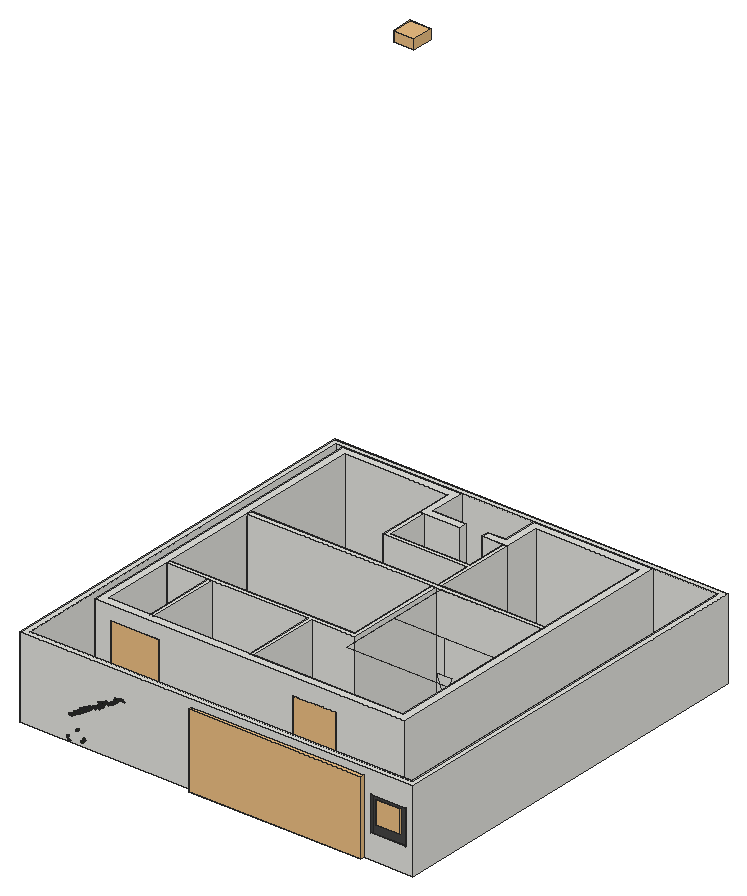
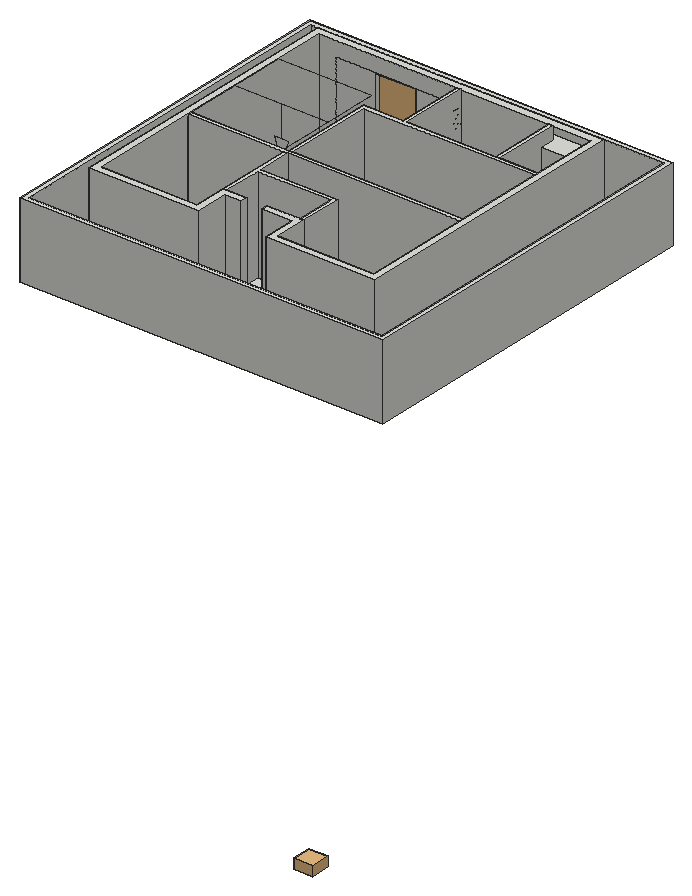
# SketchUp Ruby script. Lengths in millimetres.
U = 1.mm
M = Sketchup.active_model
def pt(a) = Geom::Point3d.new(a.map { |v| v * U })
def face(e, loops, mat)
  f = e.add_face(loops[0].map { |a| pt(a) })
  loops[1..].each { |l| e.add_face(l.map { |a| pt(a) }).erase! }
  f.material = f.back_material = mat if mat
  f
end
# faces: each face lists its corners as indices into pts; further lists are holes
def faces(e, pts, list, mat = nil) = list.each { |f| face(e, (f[0].is_a?(Array) ? f : [f]).map { |l| l.map { |i| pts[i] } }, mat) }
# xy, xz, yz: faces in a plane at the given z, y or x. An outline is a flat list of corners, or four numbers for a rectangle; further outlines are holes
def ring(l) = l.size == 4 ? [[l[0], l[1]], [l[2], l[1]], [l[2], l[3]], [l[0], l[3]]] : l.each_slice(2).to_a
def flat(e, list, mat, &to3) = list.each { |f| face(e, (f[0].is_a?(Array) ? f : [f]).map { |l| ring(l).map { |u, v| to3.(u, v) } }, mat) }
def xy(e, z, list, mat = nil) = flat(e, list, mat) { |x, y| [x, y, z] }
def xz(e, y, list, mat = nil) = flat(e, list, mat) { |x, z| [x, y, z] }
def yz(e, x, list, mat = nil) = flat(e, list, mat) { |y, z| [x, y, z] }
def lines(e, pts, list) = list.each { |a, b| e.add_line(pt(pts[a]), pt(pts[b])) }
# prism: a flat outline (further loops are holes) pulled along v
def prism(e, loops, v, mat = nil)
  f = face(e, loops, mat); d = Geom::Vector3d.new(v.map { |x| x * U })
  f.pushpull(f.normal.samedirection?(d) ? d.length : -d.length)
end
def box(e, o, s, mat = nil) = prism(e, [[o, [o[0] + s[0], o[1], o[2]], [o[0] + s[0], o[1] + s[1], o[2]], [o[0], o[1] + s[1], o[2]]]], [0, 0, s[2]], mat)
def at(x, y, z, deg = 0) = Geom::Transformation.translation(pt([x, y, z])) * Geom::Transformation.rotation(ORIGIN, Z_AXIS, deg.degrees)
def axes(o, x, y, z) = Geom::Transformation.new([*x, 0, *y, 0, *z, 0, *pt(o).to_a, 1])
def part(name) = M.definitions.add(name)
# library, detail: a bought-in or finely detailed component or shape, given as its bounding box
def library(name, o, s) = part(name).tap { |d| box(d.entities, o, s) }
def detail(e, o, s) = box(e.add_group.entities, o, s)
def put(e, d, t, mat = nil) = e.add_instance(d, t).tap { |i| i.material = mat if mat }
def group(e, t, mat = nil) = e.add_group.tap { |g| g.transformation = t; g.material = mat if mat }.entities
root = M.entities
M.materials.add("[Granite Dark Gray]").color = [69, 68, 68]
M.materials.add("efeu1").color = [18, 25, 13]
M.materials.add("efeu2").color = [43, 57, 29]
c1 = part("ivyleaf_10")
p = [[0,12.8,-0.8],[-1.5,51.3,-10.9],[-4.9,51,-11.6],[-13.6,26.5,-7.3],[-13.2,15.9,-4.6],[-21.1,19.3,-7.2],
  [-29.5,16.3,-8.3],[-29.2,8.3,-6.2],[-19.7,-9.8,0.5],[-7.6,-13,4],[1,-12.2,5.8],[-0.4,51.1,-11.1],
  [-1.5,51.1,-10.9],[1,-12.4,5.9],[16.9,-12.4,3.5],[35.1,9.1,-5.1],[35,12.9,-6.1],[20.5,16.4,-4.9],
  [15.8,15,-3.8],[15.3,27.6,-7.1],[12.8,31.3,-7.8]]
faces(c1.entities,p,[[0,1,2,3,4,5,6,7,8,9,10],[11,12,0,13,14,15,16,17,18,19,20]],"efeu2")
c2 = part("ivyleaf_9")
p = [[39.1,54.8,31.7],[34.5,51.8,30.2],[-5.3,25.2,17.3],[-17.9,28.3,20.9],[-21.6,21.7,17],[-20.2,4.3,5.3],
  [-22.9,-0.3,2.5],[-17.1,-4,-0.6],[-2,-2.1,-1.2],[-0.7,-15.4,-10.1],[16.6,-22.3,-16.7],[21.1,-15.1,-12.5],
  [32.7,-10.7,-11],[46.1,-1.8,-6.6],[30.8,11.2,3.8]]
faces(c2.entities,p,[[0,1,2,3,4,5,6,7,8,9,10,11,12,13,14]],"efeu1")
c3 = library("portao terminado by jhon",[0,-102.4,0],[4575,189.4,2762])
c4 = library("Group\#11",[0,0,0],[1682.8,214.9,2070.1])
c5 = library("ITDHP",[-33.4,-34.2,-15.9],[968.5,150,1668.6])
c6 = part("Group242\#1")
p = [[0,0,0],[0,0,-997.2],[-228.7,0,-997.2],[1488.8,-1739.7,0],[-1488.8,-1739.7,0],[1488.8,1739.7,0],
  [1488.8,0,0],[-1488.8,1739.7,0],[228.7,0,-997.2],[-1488.8,0,0],[0,0,-1614.2]]
lines(c6.entities,p,[[0,1],[1,2],[3,4],[5,6],[7,5],[1,8],[9,0],[0,6],[8,10],[4,9],[6,3],[2,10],
  [9,7]])
c7 = part("Rectangle Light\#3")
put(c7.entities,c6,at(0,0,0))
c8 = part("Group\#23")
box(c8.entities,[0,0,0],[9144,9144,101.6])
c9 = library("RAGHU   344B",[7.3,0,0],[307,195.6,25.4])
c10 = library("Dome Light\#2",[-304.8,-304.8,0],[609.6,609.6,304.8])
p = [[3261.9,2460,2644.4],[3261.9,2460,376.2],[1860.6,2460,376.2],[1860.6,2460,2644.4]]
lines(root,p,[[0,1],[2,3],[1,2]])
put(root,c1,axes([2087.5,1125.2,996.5],[1.14647,-0.14425,0.30188],[0.61451,0.08776,-0.60237],[0.16683,0.66806,0.14431]))
put(root,c1,axes([2227,1123.5,1076.7],[-1.14042,-0.39726,-0.06521],[0.10481,0.03494,-0.71894],[0.75898,-0.60174,0.0013]))
put(root,c1,axes([2487.7,1127.9,1168.1],[1.40853,-0.16077,0.0819],[0.14809,-0.0276,-0.75728],[0.30982,0.74409,-0.01039]))
put(root,c1,axes([2211.8,1127,1015.9],[1.36855,-0.00361,-0.09168],[-0.17454,-0.0063,-0.71906],[0.00529,0.72487,-0.0067]))
put(root,c1,axes([1950.7,1114.9,376.8],[0.16677,0.51977,0.47683],[0.13328,0.47171,-0.52706],[-1.3358,0.11196,0.00694]))
put(root,c2,axes([2675.6,1112.7,1367.7],[1.14223,0.42917,0.21801],[0.26909,0.1759,-0.73551],[-0.87572,0.61383,0.05835]))
put(root,c1,axes([1941.5,1127.4,839.5],[1.08139,-0.33434,0.00262],[0.02934,0.02105,-0.65876],[0.63567,0.56781,0.02596]))
put(root,c2,axes([2938.7,1117.8,1436.5],[1.15383,-0.02714,0.55158],[1.03903,0.15292,-0.59253],[-0.15844,0.80524,0.13112]))
put(root,c1,axes([1802.2,1127.3,748.7],[0.87541,-0.43119,-0.08942],[-0.10174,0.07367,-0.63024],[0.83191,0.46275,0.01702]))
put(root,c2,axes([2883.8,1117.5,1403.4],[1.44406,0.20956,0.20212],[0.37338,0.04888,-0.78715],[-0.40943,0.78369,-0.00495]))
put(root,c1,axes([2734.2,1124.8,1338.8],[-1.44401,-0.1281,-0.03694],[0.06469,0.02052,-0.76933],[0.24534,-0.75935,-0.01456]))
put(root,c1,axes([2138.7,1124.5,1019.4],[-0.75397,0.57073,-0.00023],[-0.00302,-0.00138,-0.69474],[-1.0862,-0.39616,0.00209]))
put(root,c1,axes([2245.3,1130.3,1039.4],[1.22175,0.24323,-0.15892],[-0.26862,-0.07583,-0.68618],[-0.48334,0.65696,-0.02036]))
put(root,c1,axes([2785.2,1124,1392.8],[0.87594,-0.48565,-0.40345],[-0.39684,0.35434,-0.6644],[1.13421,0.49904,0.07912]))
put(root,c1,axes([2595.6,1124.3,1225.1],[-1.31814,0.24129,0.24295],[-0.45087,0.05814,-0.73309],[-0.47053,-0.73166,0.02186]))
put(root,c1,axes([2418,1128.8,1162.7],[-1.16783,0.29379,-0.26503],[0.40269,-0.16962,-0.67789],[-0.63632,-0.64652,0.05741]))
put(root,c1,axes([2246.2,1132.2,1063.9],[0.54559,-0.61256,0.19596],[0.57494,-0.06115,-0.63309],[1.08059,0.34182,0.2379]))
put(root,c1,axes([2113,1126,187.9],[0.80503,0.17543,0.57575],[1.01265,0.21996,-0.45792],[-0.53546,0.67972,-0.00041]))
put(root,c2,axes([2651.2,1128.9,1308.3],[-0.72724,0.20612,0.62733],[-1.14354,0.19209,-0.4291],[-0.52125,-0.70899,0.06612]))
put(root,c1,axes([2290.1,1127,1106.5],[-0.78834,0.57906,-0.04144],[0.05747,-0.02934,-0.71192],[-1.10339,-0.41525,-0.00747]))
put(root,c2,axes([2593.4,1126.5,1287.1],[1.40082,-0.25988,0.08859],[0.19166,0.01971,-0.77885],[0.48614,0.74108,0.05178]))
put(root,c1,axes([1905.8,1116.9,353.5],[-0.20645,0.19287,0.66736],[-0.6237,0.58136,-0.22129],[-1.16574,-0.3452,0.0002]))
put(root,c1,axes([2376.5,1125.8,1120.4],[0.41629,0.67018,0.1664],[0.02658,0.17022,-0.70392],[-1.31394,0.21577,0.03848]))
put(root,c1,axes([2077.2,1130.6,100.3],[-1.20166,-0.34105,0.12031],[-0.20148,-0.05716,-0.71762],[0.65815,-0.64021,-0.00002]))
put(root,c2,axes([3074.3,1117.4,1564],[-0.14401,0.62355,0.52426],[-0.5244,0.47589,-0.60579],[-1.45907,-0.23258,0.16598]))
put(root,c1,axes([2083.8,1127.2,985.5],[-0.9922,-0.29503,-0.33284],[0.58225,0.13437,-0.5983],[0.61443,-0.60375,0.02949]))
put(root,c1,axes([1847.2,1134.9,825.7],[0.26434,0.55426,-0.30055],[-0.38483,-0.25234,-0.5588],[-1.13659,0.21434,0.1193]))
put(root,c1,axes([2033.8,1132.8,966.4],[1.20012,-0.23106,-0.15832],[-0.28876,0.04606,-0.67153],[0.4481,0.64852,-0.00872]))
put(root,c2,axes([2529.7,1141.6,1158.8],[0.17517,-0.73,0.19546],[0.26456,-0.17719,-0.72723],[1.41374,0.12361,0.11187]))
put(root,c1,axes([1701.9,1128.5,6.6],[0.41838,-0.09412,-0.61048],[-1.06203,0.2476,-0.23911],[0.50409,0.59975,0.00292]))
put(root,c1,axes([2611,1128.2,1269.6],[0.17115,0.74499,0.07381],[-0.06511,0.07835,-0.74915],[-1.42331,0.086,0.04314]))
put(root,c1,axes([2156.7,1130.4,990.8],[-1.12894,-0.39996,-0.06692],[0.11408,0.0308,-0.71538],[0.7633,-0.59615,0.00794]))
put(root,c2,axes([2648.4,1126.8,1311.5],[1.39789,-0.11145,-0.17675],[-0.32698,0.04555,-0.74266],[0.22635,0.75409,0.01873]))
put(root,c1,axes([3086.7,1129.5,1527.5],[-0.87891,-0.62071,-0.33517],[0.63358,0.16142,-0.75763],[1.18365,-0.54731,0.15666]))
put(root,c1,axes([2872.3,1134.5,1396.1],[-1.18913,-0.46802,0.23312],[-0.38278,-0.12017,-0.78031],[0.91856,-0.65596,-0.02338]))
put(root,c2,axes([2527,1140.2,1184.9],[-1.4479,-0.0903,-0.02056],[0.03876,0.00287,-0.76611],[0.17195,-0.76105,-0.00045]))
put(root,c2,axes([2684.4,1124.5,1319.4],[1.0942,0.49964,-0.08552],[-0.12552,-0.05449,-0.76169],[-0.95654,0.57869,0.00212]))
put(root,c1,axes([2166.9,1133.9,982.2],[1.20048,0.27627,0.02283],[0.00864,0.04644,-0.68742],[-0.52752,0.62947,0.0407]))
put(root,c2,axes([2611.2,1131.1,1219.3],[1.29213,-0.19777,0.3143],[0.62228,0.00788,-0.70133],[0.33504,0.7481,0.09048]))
put(root,c1,axes([1641.3,1125,74.3],[0.34683,0.44503,-0.4286],[0.28466,0.40179,0.48079],[1.14094,-0.23553,0.01033]))
put(root,c1,axes([2002.9,1136.6,906.3],[-0.1027,-0.66383,0.00555],[0.02053,-0.00644,-0.66592],[1.26328,-0.05386,0.01127]))
put(root,c1,axes([2344.7,1133.8,1092.8],[-1.26781,0.26235,0.00767],[-0.08042,-0.08656,-0.70948],[-0.49299,-0.66054,0.09602]))
put(root,c2,axes([2711.4,1125.1,1339.7],[0.66533,0.6864,-0.0181],[-0.03371,-0.01129,-0.77022],[-1.30637,0.34987,0.01066]))
put(root,c1,axes([1798,1141.1,753.8],[-0.57971,-0.53097,0.24391],[-0.25724,-0.20357,-0.61196],[1.0819,-0.33291,-0.01481]))
put(root,c1,axes([1741.7,1141.3,714.9],[-0.79482,-0.37017,0.33114],[-0.4073,-0.2563,-0.55642],[0.853,-0.4673,0.04287]))
put(root,c1,axes([2265.9,1134.2,1011.5],[1.03278,-0.19104,-0.4391],[-0.69613,0.26296,-0.56643],[0.58821,0.64663,0.10062]))
put(root,c1,axes([1952.8,1141.9,831.4],[0.77305,-0.50539,0.20075],[0.36414,-0.10173,-0.64323],[0.96878,0.44152,0.08159]))
put(root,c1,axes([2042.8,1138.8,920.3],[1.13684,0.31347,-0.01678],[-0.02813,-0.00794,-0.67459],[-0.59678,0.59751,-0.00017]))
put(root,c1,axes([2092.9,1138.9,946.1],[0.83948,0.51607,-0.0565],[-0.04985,-0.05192,-0.67875],[-0.98679,0.44165,-0.01377]))
put(root,c1,axes([2204.8,1132.1,1024.1],[0.3654,0.63545,0.29134],[0.17355,0.27678,-0.66379],[-1.31907,0.21244,-0.00663]))
put(root,c1,axes([2055.9,1138.4,910.8],[-1.19265,0.24212,0.03133],[-0.14567,-0.11287,-0.65856],[-0.44123,-0.6172,0.13272]))
put(root,c1,axes([1663.3,1133.7,111.6],[0.44207,-0.21789,-0.57506],[-0.83258,0.37348,-0.31821],[0.82255,0.49513,-0.01304]))
put(root,c1,axes([2184,1137.8,965.5],[-1.33928,-0.07647,-0.06876],[0.13459,-0.01463,-0.7075],[0.14209,-0.7069,0.02208]))
put(root,c2,axes([2576.4,1144.7,1209.1],[-1.10889,0.13379,0.48618],[-0.95061,-0.05123,-0.5845],[-0.13163,-0.75711,0.12546]))
put(root,c1,axes([1961.4,1140.4,834.8],[-0.51233,-0.62282,-0.03193],[0.02408,0.02931,-0.6785],[1.18666,-0.26949,-0.00002]))
put(root,c1,axes([1861.6,1143.6,765.7],[0.11262,-0.65084,0.09162],[0.22553,-0.07991,-0.64425],[1.23039,0.07422,0.1097]))
put(root,c1,axes([2100.5,1135.7,963.8],[0.35088,-0.56899,-0.32951],[-0.03237,0.33797,-0.59313],[1.25097,0.16834,0.07707]))
put(root,c1,axes([1912.8,1138.8,840],[-0.41835,0.63903,-0.06258],[0.06384,-0.05463,-0.67563],[-1.22034,-0.22192,-0.01389]))
put(root,c1,axes([2037.2,1142.3,912.8],[0.57227,0.59214,-0.09712],[-0.05534,-0.09412,-0.6639],[-1.14067,0.30164,-0.01651]))
put(root,c2,axes([3216.3,1134.5,1584.3],[1.60333,-0.08607,0.1036],[0.21434,0.09021,-0.84085],[0.14061,0.84398,0.10044]))
put(root,c1,axes([1722.1,1142.7,720],[-0.8891,0.41506,-0.1659],[0.07984,-0.1982,-0.614],[-0.84695,-0.4544,0.11628]))
put(root,c1,axes([1683.5,1143.9,697.5],[0.99386,-0.3603,0.08583],[0.24125,0.03446,-0.6266],[0.66235,0.52809,0.09944]))
put(root,c2,axes([2651.4,1144.5,1255.4],[-1.39761,0.26588,-0.01109],[0.0257,0.00473,-0.78095],[-0.50582,-0.73442,-0.00904]))
put(root,c1,axes([1964.2,1144.3,820.5],[1.28133,-0.01571,0.05918],[0.11272,0.0013,-0.67343],[0.02957,0.67584,0.00267]))
put(root,c1,axes([2250.9,1137.8,1058.7],[0.64921,0.57335,0.2312],[0.17275,0.21475,-0.66647],[-1.16383,0.3517,0.03005]))
put(root,c1,axes([2340.8,1137.4,1100.2],[-0.18264,-0.02984,0.71109],[1.1457,0.37938,0.09716],[-0.72261,0.60904,-0.02568]))
put(root,c1,axes([2011.3,1139.5,905.1],[-0.72427,0.20234,0.54537],[-1.03186,0.11275,-0.42015],[-0.40112,-0.65539,0.09609]))
put(root,c1,axes([2924.7,1136.7,1429.1],[-0.60924,0.68131,0.32435],[-0.41882,0.25272,-0.74804],[-1.37368,-0.37922,0.08422]))
put(root,c1,axes([2433.8,1146.8,1120],[-1.05987,0.38935,-0.31691],[0.39921,-0.24955,-0.67519],[-0.86806,-0.59015,0.07643]))
put(root,c1,axes([2223.4,1143.2,989.3],[-1.00531,-0.4412,-0.21337],[0.4215,0.06495,-0.68259],[0.83205,-0.56597,0.08799]))
put(root,c1,axes([1910.2,1143.8,787],[-0.48525,-0.47153,0.39714],[0.78354,0.18966,0.48949],[-0.87334,0.43215,0.2185]))
put(root,c1,axes([2311.9,1144.4,1047.3],[-1.34262,-0.1772,0.10149],[-0.18137,-0.03717,-0.72726],[0.34374,-0.71175,0.01271]))
put(root,c1,axes([2590.6,1146,1201.5],[1.28279,0.30834,0.20555],[0.36073,0.07976,-0.74117],[-0.60603,0.70013,-0.00609]))
put(root,c1,axes([1960.7,1137.6,858.3],[0.32576,-0.02559,-0.66433],[-0.78395,0.53438,-0.12671],[0.99317,0.4302,0.11788]))
put(root,c1,axes([1982.9,1149.2,825.1],[1.28689,0.00904,0.05914],[0.11267,-0.0039,-0.67621],[-0.01649,0.67874,-0.00467]))
put(root,c1,axes([1833.5,1146.4,784],[-0.83766,0.46308,-0.00992],[0.01893,-0.00423,-0.63886],[-0.88134,-0.44023,-0.00429]))
put(root,c1,axes([2295.7,1148.4,1017.4],[0.80941,-0.58283,0.08136],[-0.11218,0.05769,0.72137],[-1.11436,-0.42914,-0.01353]))
put(root,c2,axes([2617.5,1141.4,1240.2],[1.41382,0.20155,-0.1232],[-0.2359,-0.01349,-0.76948],[-0.3827,0.75289,0.0192]))
put(root,c1,axes([3173.9,1150.6,1595.6],[1.4026,0.42686,0.03072],[0.02869,0.03524,-0.85136],[-0.814,0.73677,0.02292]))
put(root,c1,axes([2347.6,1150.4,1054.1],[0.14125,0.72377,-0.09823],[-0.51469,-0.06449,-0.67949],[-1.29131,0.10487,0.26009]))
put(root,c1,axes([1976.8,1151,841.1],[0.13058,0.67305,-0.08399],[-0.0077,-0.08401,-0.67652],[-1.29086,0.06859,-0.00446]))
put(root,c1,axes([1837.1,1161.2,758.5],[-0.6104,-0.37581,0.43332],[-0.04619,-0.48712,-0.44044],[1.09066,-0.23096,0.22386]))
put(root,c2,axes([2919,1151.2,1418.9],[1.34132,-0.40615,-0.05695],[-0.11526,0.00892,-0.81312],[0.77199,0.70701,-0.02246]))
put(root,c1,axes([2830.5,1140.4,1345.8],[0.00272,-0.01779,0.80228],[0.68542,0.71696,0.01526],[-1.36483,0.36003,0.00926]))
put(root,c1,axes([1732.9,1151.8,684.4],[-0.85829,-0.22462,-0.39564],[0.78116,0.03946,-0.49025],[0.37355,-0.59863,0.11614]))
put(root,c1,axes([3030.4,1151.4,1506],[-1.53799,0.1931,-0.06685],[0.11701,-0.03029,-0.83072],[-0.37088,-0.8103,0.01512]))
put(root,c1,axes([1774.7,1152.8,716.1],[-1.16417,0.19732,0.08542],[-0.16731,0.00557,-0.64237],[-0.37346,-0.6176,0.0215]))
put(root,c1,axes([2493.6,1155,1170.6],[-1.29549,0.31597,-0.11703],[0.1969,-0.05507,-0.75042],[-0.61029,-0.68848,0.00631]))
put(root,c1,axes([3056.5,1155.1,1512.6],[-1.57039,-0.071,-0.10658],[0.20404,-0.00285,-0.82809],[0.13331,-0.83198,0.01193]))
put(root,c1,axes([2113.4,1156.8,912.6],[1.1383,-0.03936,-0.35907],[-0.64946,0.16622,-0.58662],[0.22547,0.67751,0.12306]))
put(root,c1,axes([2048.9,1158.8,879.4],[1.28694,0.08427,-0.10291],[-0.20899,0.05281,-0.6783],[-0.14286,0.68194,0.06524]))
put(root,c1,axes([1976.3,1163.9,842.3],[-1.14856,0.29947,0.08062],[-0.16168,0.01002,-0.6731],[-0.56767,-0.60877,0.02858]))
put(root,c1,axes([1733.2,1165,691.6],[-0.60057,0.55437,-0.02515],[0.03922,-0.01721,-0.63782],[-1.05543,-0.31609,-0.00939]))
put(root,c2,axes([2574.4,1157.2,1220.3],[1.14365,0.46244,0.13789],[0.15892,0.11725,-0.75712],[-0.90455,0.60527,0.04132]))
put(root,c2,axes([2624.1,1157.6,1238.1],[0.80785,0.59559,0.25643],[0.26398,0.216,-0.73128],[-1.20557,0.4464,0.01171]))
put(root,c3,axes([5232.4,1226.8,-101.6],[1.10738,0,0],[0,1,0],[0,0,0.78614]))
put(root,c4,axes([7229.2,2446,210.4],[0.74576,0,0],[0,0.57,0],[0,0,1.13036]))
put(root,c5,axes([1909.4,2477.6,384.8],[1.44679,0,0],[0,0.92467,0],[0,0,1.35933]))
g1 = group(root,at(2833.1,2674.6,0))
xy(g1,0,[[0,0,127,2133.6]])
xy(g1,3048,[[0,0,127,2133.6]])
xz(g1,2133.6,[[0,0,127,3048]])
yz(g1,0,[[0,0,2133.6,3048]])
yz(g1,127,[[0,0,2133.6,3048]])
g2 = group(root,at(1613.9,2674.6,0))
prism(g2,[[[5562.6,5105.4,0],[5562.6,2133.6,0],[4292.6,2133.6,0],[4292.6,0,0],[4165.6,0,0],[4165.6,2133.6,0],[1346.2,2133.6,0],[1219.2,2133.6,0],[0,2133.6,0],[0,2260.6,0],[5435.6,2260.6,0],[5435.6,5105.4,0]]],[0,0,3048])
put(root,c7,at(8812,6040.4,3047.7))
put(root,c8,at(1385.3,2446,-101.6))
g3 = group(root,at(1385.3,2446,0))
xy(g3,0,[[0,0,0,9144,3500.3,9144,3500.3,8102.6,4459.1,8102.6,4459.1,7874,3276.6,7874,3276.6,8915.4,228.6,8915.4,228.6,228.6,8915.4,228.6,8915.4,8915.4,5867.4,8915.4,5867.4,7874,5119.1,7874,5119.1,8102.6,5638.8,8102.6,5638.8,9144,9144,9144,9144,0]])
xy(g3,210.4,[[5838.3,0,7098.8,228.6]])
xy(g3,288,[[4394.2,228.6,4521.2,579.4]])
xy(g3,376.3,[[475.3,0,1877,723.9]])
xy(g3,2548.8,[[5838.3,0,7098.8,228.6]])
xy(g3,2564.5,[[4394.2,228.6,4521.2,579.4]])
xy(g3,2644.4,[[475.3,0,1877,723.9]])
xy(g3,3048,[[0,0,9144,0,9144,9144,5638.8,9144,5638.8,8102.6,5119.1,8102.6,5119.1,7874,5867.4,7874,5867.4,8915.4,8915.4,8915.4,8915.4,228.6,228.6,228.6,228.6,8915.4,3276.6,8915.4,3276.6,7874,4459.1,7874,4459.1,8102.6,3500.3,8102.6,3500.3,9144,0,9144]])
xz(g3,0,[[[0,0,9144,3048],[475.3,376.3,1877,2644.4],[5838.3,210.4,7098.8,2548.8]]])
xz(g3,228.6,[[1447.8,0,1574.8,3048],[4394.2,0,4521.2,288],[4521.2,0,4521.2,288,5838.3,288,5838.3,210.4,7098.8,210.4,7098.8,288,8374.6,288,8374.6,2564.5,4521.2,2564.5,4521.2,3048,8915.4,3048,8915.4,0],[4394.2,288,4521.2,2564.5],[4521.2,288,4521.2,2564.5,8374.6,2564.5,8374.6,288,7098.8,288,7098.8,2548.8,5838.3,2548.8,5838.3,288],
  [4394.2,2564.5,4521.2,3048]])
xz(g3,579.4,[[4394.2,288,4521.2,2564.5]])
xz(g3,723.9,[[475.3,376.3,1877,2644.4]])
xz(g3,7874,[[3276.6,0,3403.6,3048],[3403.6,0,4459.1,3048],[5119.1,0,5740.4,3048],[5740.4,0,5867.4,3048]])
xz(g3,8102.6,[[3500.3,0,4459.1,3048],[5119.1,0,5638.8,3048]])
xz(g3,8915.4,[[228.6,0,3276.6,3048],[5867.4,0,8915.4,3048]])
xz(g3,9144,[[0,0,3500.3,3048],[5638.8,0,9144,3048]])
yz(g3,0,[[0,0,9144,3048]])
yz(g3,228.6,[[228.6,0,2362.2,3048],[2362.2,0,2489.2,3048],[2489.2,0,5334,3048],[5334,0,5461,3048],[5461,0,8915.4,3048]])
yz(g3,475.3,[[0,376.3,723.9,2644.4]])
yz(g3,1877,[[0,376.3,723.9,2644.4]])
yz(g3,3276.6,[[7874,0,8915.4,3048]])
yz(g3,3500.3,[[8102.6,0,9144,3048]])
yz(g3,4394.2,[[228.6,288,579.4,2564.5]])
yz(g3,4459.1,[[7874,0,8102.6,3048]])
yz(g3,4521.2,[[228.6,288,579.4,2564.5]])
yz(g3,5119.1,[[7874,0,8102.6,3048]])
yz(g3,5638.8,[[8102.6,0,9144,3048]])
yz(g3,5838.3,[[0,210.4,228.6,2548.8]])
yz(g3,5867.4,[[7874,0,8915.4,3048]])
yz(g3,7098.8,[[0,210.4,228.6,2548.8]])
yz(g3,8915.4,[[228.6,0,5334,3048],[5334,0,5461,3048],[5461,0,8915.4,3048]])
yz(g3,9144,[[0,0,9144,3048]])
g4 = group(root,at(166.1,1226.8,-101.6))
xy(g4,0,[[5066.3,0,10132.5,152.4],[152.4,152.4,11430,11430]])
xy(g4,699.8,[[10341.4,0,11378.1,52.4]])
xy(g4,1736.4,[[10341.4,0,11378.1,52.4]])
xy(g4,2171.3,[[5312.6,0,9931.5,152.4]])
xy(g4,2389.2,[[[0,0,11582.4,11582.4],[152.4,152.4,11430,11430]]])
xz(g4,0,[[[0,0,5066.3,0,5066.3,1925,5073.1,2000.2,5093.6,2061.8,5127.8,2109.7,5175.8,2143.9,5237.3,2164.5,5312.6,2171.3,9931.5,2171.3,9992.9,2165.7,10043.2,2149,10082.3,2121.1,10110.2,2082,10126.9,2031.7,10132.5,1970.3,10132.5,0,11582.4,0,11582.4,2389.2,0,2389.2],[10341.4,699.8,11378.1,1736.4]]])
xz(g4,52.4,[[10341.4,699.8,11378.1,1736.4]],"[Granite Dark Gray]")
xz(g4,152.4,[[152.4,0,152.4,2389.2,10132.5,2389.2,10132.5,2171.3,5312.6,2171.3,5237.3,2164.5,5175.8,2143.9,5127.8,2109.7,5093.6,2061.8,5073.1,2000.2,5066.3,1925,5066.3,0],[10132.5,0,11430,2389.2],[10132.5,1970.3,10126.9,2031.7,10110.2,2082,10082.3,2121.1,10043.2,2149,9992.9,2165.7,9931.5,2171.3,10132.5,2171.3]])
xz(g4,11430,[[152.4,0,11430,2389.2]])
xz(g4,11582.4,[[0,0,11582.4,2389.2]])
yz(g4,0,[[0,0,11582.4,2389.2]])
yz(g4,152.4,[[152.4,0,11430,2389.2]])
yz(g4,5066.3,[[0,0,152.4,1925]])
yz(g4,10132.5,[[0,0,152.4,1970.3]])
yz(g4,10341.4,[[0,699.8,52.4,1736.4]],"[Granite Dark Gray]")
yz(g4,11378.1,[[0,699.8,52.4,1736.4]],"[Granite Dark Gray]")
yz(g4,11430,[[152.4,0,11430,2389.2]])
yz(g4,11582.4,[[0,0,11582.4,2389.2]])
p = [[5066.3,0,1925],[5066.3,152.4,1925],[5073.1,152.4,2000.2],[5073.1,0,2000.2],[10126.9,0,2031.7],[10126.9,152.4,2031.7],
  [10132.5,152.4,1970.3],[10132.5,0,1970.3],[5093.6,152.4,2061.8],[5093.6,0,2061.8],[10110.2,0,2082],[10110.2,152.4,2082],
  [5127.8,152.4,2109.7],[5127.8,0,2109.7],[10082.3,0,2121.1],[10082.3,152.4,2121.1],[5175.8,152.4,2143.9],[5175.8,0,2143.9],
  [10043.2,0,2149],[10043.2,152.4,2149],[5237.3,152.4,2164.5],[5237.3,0,2164.5],[9992.9,0,2165.7],[9992.9,152.4,2165.7],
  [5312.6,152.4,2171.3],[5312.6,0,2171.3],[9931.5,0,2171.3],[9931.5,152.4,2171.3]]
faces(g4,p,[[0,1,2,3],[4,5,6,7],[3,2,8,9],[10,11,5,4],[9,8,12,13],[14,15,11,10],[13,12,16,17],[18,19,15,14],
  [17,16,20,21],[22,23,19,18],[21,20,24,25],[26,27,23,22]])
put(g4,c9,axes([10457.4,52.4,964],[2.282,0,0],[0,0,3.36],[0,-1,0]))
g5 = group(root,at(1613.9,7780,0))
prism(g5,[[[5562.6,0,0],[5435.6,0,0],[0,0,0],[0,127,0],[5511.8,127,0],[5638.8,127,0],[8686.8,127,0],[8686.8,0,0]]],[0,0,3048])
g6 = group(root,at(4661.9,7907,0))
prism(g6,[[[2463.8,0,0],[2463.8,1066.8,0],[0,1066.8,0],[0,2413,0],[127,2413,0],[127,1193.8,0],[2463.8,1193.8,0],[2463.8,2413,0],[2590.8,2413,0],[2590.8,0,0]]],[0,0,3048])
put(root,c10,at(-12667.4,31714.5,0))
